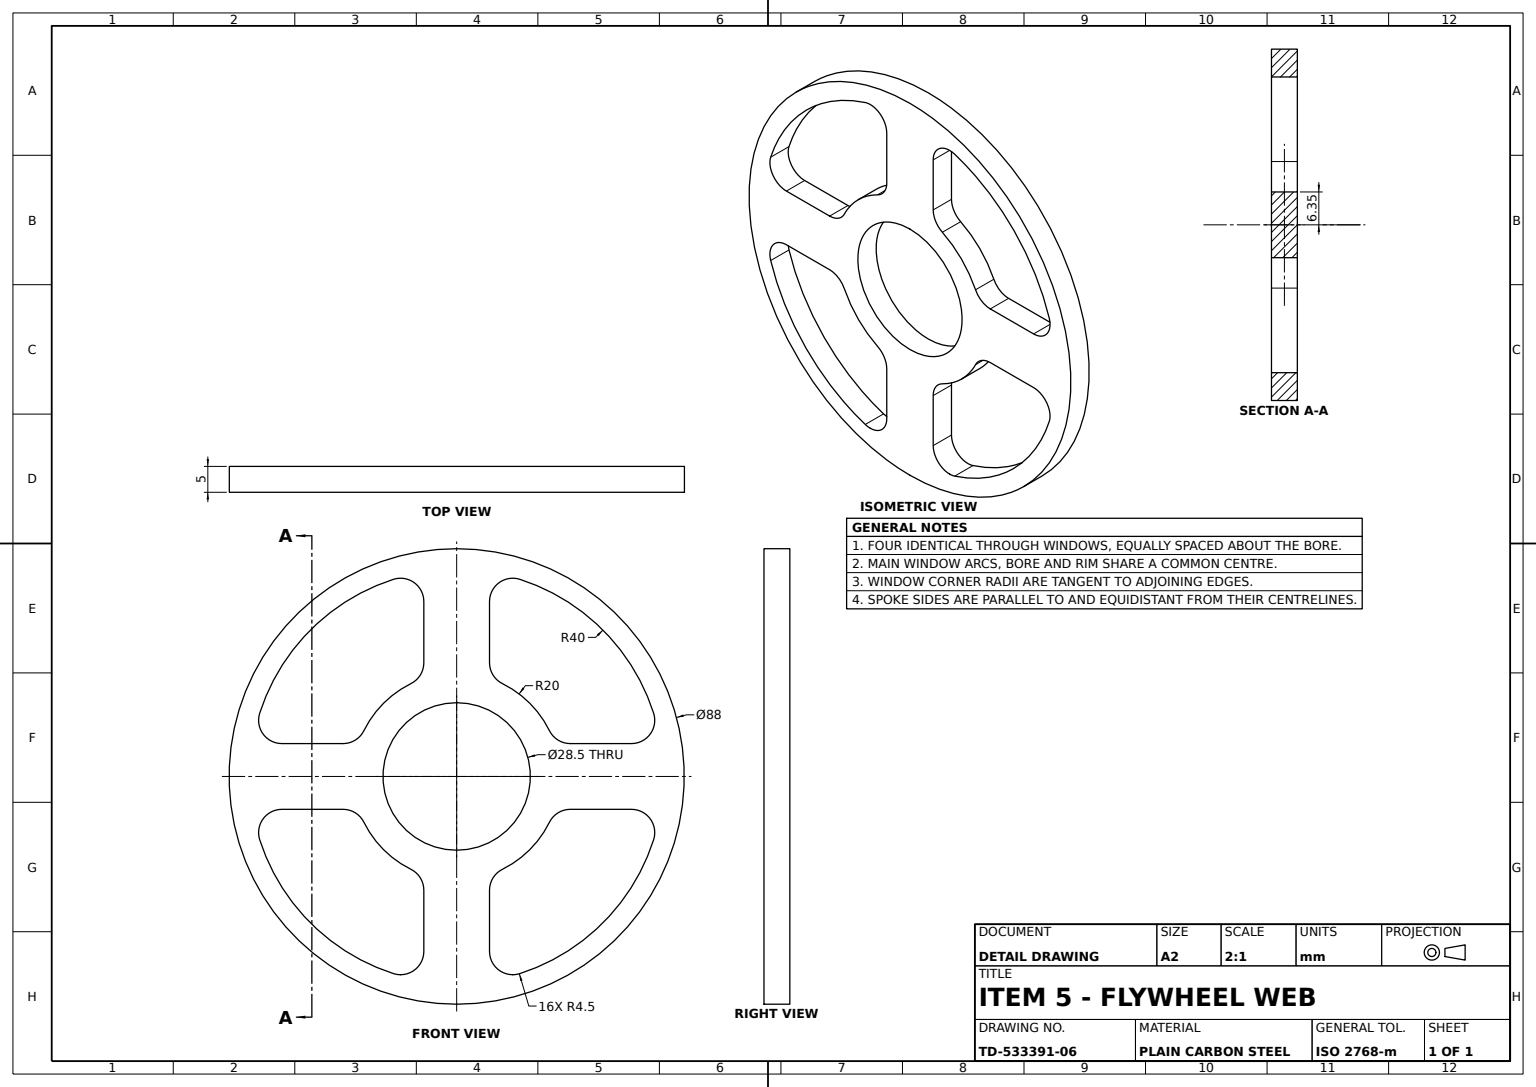
ISO-10303-21;
HEADER;
FILE_DESCRIPTION((''),'2;1');
FILE_NAME('','',(''),(''),'','','');
FILE_SCHEMA(('AUTOMOTIVE_DESIGN'));
ENDSEC;
DATA;
#1=APPLICATION_CONTEXT('');
#2=PRODUCT_CONTEXT('',#1,'mechanical');
#3=PRODUCT('','','',(#2));
#4=PRODUCT_DEFINITION_FORMATION('','',#3);
#5=PRODUCT_DEFINITION_CONTEXT('',#1,'design');
#6=PRODUCT_DEFINITION('','',#4,#5);
#7=PRODUCT_DEFINITION_SHAPE('','',#6);
#8=(LENGTH_UNIT()NAMED_UNIT(*)SI_UNIT(.MILLI.,.METRE.));
#9=(NAMED_UNIT(*)PLANE_ANGLE_UNIT()SI_UNIT($,.RADIAN.));
#10=(NAMED_UNIT(*)SI_UNIT($,.STERADIAN.)SOLID_ANGLE_UNIT());
#11=UNCERTAINTY_MEASURE_WITH_UNIT(LENGTH_MEASURE(1.E-05),#8,'distance_accuracy_value','');
#12=(GEOMETRIC_REPRESENTATION_CONTEXT(3)GLOBAL_UNCERTAINTY_ASSIGNED_CONTEXT((#11))GLOBAL_UNIT_ASSIGNED_CONTEXT((#8,#9,#10))REPRESENTATION_CONTEXT('',''));
#13=CARTESIAN_POINT('',(12.225352,0.,38.085965));
#14=VERTEX_POINT('',#13);
#15=CARTESIAN_POINT('',(12.225352,5.,38.085965));
#16=VERTEX_POINT('',#15);
#17=CARTESIAN_POINT('',(12.225352,-39.,38.085965));
#18=DIRECTION('',(0.,1.,0.));
#19=VECTOR('',#18,1000.);
#20=LINE('',#17,#19);
#21=EDGE_CURVE('',#14,#16,#20,.T.);
#22=ORIENTED_EDGE('',*,*,#21,.T.);
#23=CARTESIAN_POINT('',(38.085965,5.,12.225352));
#24=VERTEX_POINT('',#23);
#25=CARTESIAN_POINT('',(0.,5.,0.));
#26=DIRECTION('',(0.,0.,1.));
#27=AXIS2_PLACEMENT_3D('',#25,#18,#26);
#28=CIRCLE('',#27,40.);
#29=EDGE_CURVE('',#16,#24,#28,.T.);
#30=ORIENTED_EDGE('',*,*,#29,.T.);
#31=CARTESIAN_POINT('',(38.085965,0.,12.225352));
#32=VERTEX_POINT('',#31);
#33=CARTESIAN_POINT('',(38.085965,-39.,12.225352));
#34=LINE('',#33,#19);
#35=EDGE_CURVE('',#32,#24,#34,.T.);
#36=ORIENTED_EDGE('',*,*,#35,.F.);
#37=CARTESIAN_POINT('',(0.,0.,0.));
#38=AXIS2_PLACEMENT_3D('',#37,#18,#26);
#39=CIRCLE('',#38,40.);
#40=EDGE_CURVE('',#14,#32,#39,.T.);
#41=ORIENTED_EDGE('',*,*,#40,.F.);
#42=EDGE_LOOP('',(#22,#30,#36,#41));
#43=FACE_OUTER_BOUND('',#42,.T.);
#44=CARTESIAN_POINT('',(0.,-39.,0.));
#45=AXIS2_PLACEMENT_3D('',#44,#18,#26);
#46=CYLINDRICAL_SURFACE('',#45,40.);
#47=ADVANCED_FACE('',(#43),#46,.F.);
#48=CARTESIAN_POINT('',(0.,5.,-44.));
#49=VERTEX_POINT('',#48);
#50=CARTESIAN_POINT('',(0.,0.,-44.));
#51=VERTEX_POINT('',#50);
#52=DIRECTION('',(0.,-1.,0.));
#53=VECTOR('',#52,1000.);
#54=LINE('',#48,#53);
#55=EDGE_CURVE('',#49,#51,#54,.T.);
#56=ORIENTED_EDGE('',*,*,#55,.F.);
#57=CARTESIAN_POINT('',(0.,5.,44.));
#58=VERTEX_POINT('',#57);
#59=CIRCLE('',#27,44.);
#60=EDGE_CURVE('',#58,#49,#59,.T.);
#61=ORIENTED_EDGE('',*,*,#60,.F.);
#62=CARTESIAN_POINT('',(0.,0.,44.));
#63=VERTEX_POINT('',#62);
#64=LINE('',#57,#53);
#65=EDGE_CURVE('',#58,#63,#64,.T.);
#66=ORIENTED_EDGE('',*,*,#65,.T.);
#67=CIRCLE('',#38,44.);
#68=EDGE_CURVE('',#63,#51,#67,.T.);
#69=ORIENTED_EDGE('',*,*,#68,.T.);
#70=EDGE_LOOP('',(#56,#61,#66,#69));
#71=FACE_OUTER_BOUND('',#70,.T.);
#72=DIRECTION('',(0.,0.,-1.));
#73=AXIS2_PLACEMENT_3D('',#25,#52,#72);
#74=CYLINDRICAL_SURFACE('',#73,44.);
#75=ADVANCED_FACE('',(#71),#74,.T.);
#76=CARTESIAN_POINT('',(10.85,0.,38.301294));
#77=VERTEX_POINT('',#76);
#78=CARTESIAN_POINT('',(10.85,5.,38.301294));
#79=VERTEX_POINT('',#78);
#80=CARTESIAN_POINT('',(10.85,-39.,38.301294));
#81=LINE('',#80,#19);
#82=EDGE_CURVE('',#77,#79,#81,.T.);
#83=ORIENTED_EDGE('',*,*,#82,.T.);
#84=CARTESIAN_POINT('',(10.85,5.,33.801294));
#85=AXIS2_PLACEMENT_3D('',#84,#18,#26);
#86=CIRCLE('',#85,4.5);
#87=EDGE_CURVE('',#79,#16,#86,.T.);
#88=ORIENTED_EDGE('',*,*,#87,.T.);
#89=ORIENTED_EDGE('',*,*,#21,.F.);
#90=CARTESIAN_POINT('',(10.85,0.,33.801294));
#91=AXIS2_PLACEMENT_3D('',#90,#18,#26);
#92=CIRCLE('',#91,4.5);
#93=EDGE_CURVE('',#77,#14,#92,.T.);
#94=ORIENTED_EDGE('',*,*,#93,.F.);
#95=EDGE_LOOP('',(#83,#88,#89,#94));
#96=FACE_OUTER_BOUND('',#95,.T.);
#97=CARTESIAN_POINT('',(10.85,-39.,33.801294));
#98=AXIS2_PLACEMENT_3D('',#97,#18,#26);
#99=CYLINDRICAL_SURFACE('',#98,4.5);
#100=ADVANCED_FACE('',(#96),#99,.F.);
#101=CARTESIAN_POINT('',(-8.857143,0.,17.931844));
#102=VERTEX_POINT('',#101);
#103=CARTESIAN_POINT('',(-8.857143,5.,17.931844));
#104=VERTEX_POINT('',#103);
#105=CARTESIAN_POINT('',(-8.857143,-39.,17.931844));
#106=LINE('',#105,#19);
#107=EDGE_CURVE('',#102,#104,#106,.T.);
#108=ORIENTED_EDGE('',*,*,#107,.F.);
#109=CARTESIAN_POINT('',(-6.35,0.,21.966509));
#110=VERTEX_POINT('',#109);
#111=CARTESIAN_POINT('',(-10.85,0.,21.966509));
#112=AXIS2_PLACEMENT_3D('',#111,#18,#26);
#113=CIRCLE('',#112,4.5);
#114=EDGE_CURVE('',#110,#102,#113,.T.);
#115=ORIENTED_EDGE('',*,*,#114,.F.);
#116=CARTESIAN_POINT('',(-6.35,5.,21.966509));
#117=VERTEX_POINT('',#116);
#118=CARTESIAN_POINT('',(-6.35,-39.,21.966509));
#119=LINE('',#118,#19);
#120=EDGE_CURVE('',#110,#117,#119,.T.);
#121=ORIENTED_EDGE('',*,*,#120,.T.);
#122=CARTESIAN_POINT('',(-10.85,5.,21.966509));
#123=AXIS2_PLACEMENT_3D('',#122,#18,#26);
#124=CIRCLE('',#123,4.5);
#125=EDGE_CURVE('',#117,#104,#124,.T.);
#126=ORIENTED_EDGE('',*,*,#125,.T.);
#127=EDGE_LOOP('',(#108,#115,#121,#126));
#128=FACE_OUTER_BOUND('',#127,.T.);
#129=CARTESIAN_POINT('',(-10.85,-39.,21.966509));
#130=AXIS2_PLACEMENT_3D('',#129,#18,#26);
#131=CYLINDRICAL_SURFACE('',#130,4.5);
#132=ADVANCED_FACE('',(#128),#131,.F.);
#133=CARTESIAN_POINT('',(-17.931844,0.,8.857143));
#134=VERTEX_POINT('',#133);
#135=CIRCLE('',#38,20.);
#136=EDGE_CURVE('',#134,#102,#135,.T.);
#137=ORIENTED_EDGE('',*,*,#136,.F.);
#138=CARTESIAN_POINT('',(-21.966509,0.,6.35));
#139=VERTEX_POINT('',#138);
#140=CARTESIAN_POINT('',(-21.966509,0.,10.85));
#141=AXIS2_PLACEMENT_3D('',#140,#18,#26);
#142=CIRCLE('',#141,4.5);
#143=EDGE_CURVE('',#134,#139,#142,.T.);
#144=ORIENTED_EDGE('',*,*,#143,.T.);
#145=CARTESIAN_POINT('',(-33.801294,0.,6.35));
#146=VERTEX_POINT('',#145);
#147=CARTESIAN_POINT('',(0.,0.,6.35));
#148=DIRECTION('',(-1.,0.,0.));
#149=VECTOR('',#148,1000.);
#150=LINE('',#147,#149);
#151=EDGE_CURVE('',#139,#146,#150,.T.);
#152=ORIENTED_EDGE('',*,*,#151,.T.);
#153=CARTESIAN_POINT('',(-38.085965,0.,12.225352));
#154=VERTEX_POINT('',#153);
#155=CARTESIAN_POINT('',(-33.801294,0.,10.85));
#156=AXIS2_PLACEMENT_3D('',#155,#18,#26);
#157=CIRCLE('',#156,4.5);
#158=EDGE_CURVE('',#146,#154,#157,.T.);
#159=ORIENTED_EDGE('',*,*,#158,.T.);
#160=CARTESIAN_POINT('',(-12.225352,0.,38.085965));
#161=VERTEX_POINT('',#160);
#162=EDGE_CURVE('',#154,#161,#39,.T.);
#163=ORIENTED_EDGE('',*,*,#162,.T.);
#164=CARTESIAN_POINT('',(-10.85,0.,38.301294));
#165=VERTEX_POINT('',#164);
#166=CARTESIAN_POINT('',(-10.85,0.,33.801294));
#167=AXIS2_PLACEMENT_3D('',#166,#18,#26);
#168=CIRCLE('',#167,4.5);
#169=EDGE_CURVE('',#161,#165,#168,.T.);
#170=ORIENTED_EDGE('',*,*,#169,.T.);
#171=CARTESIAN_POINT('',(-6.35,0.,33.801294));
#172=VERTEX_POINT('',#171);
#173=EDGE_CURVE('',#165,#172,#168,.T.);
#174=ORIENTED_EDGE('',*,*,#173,.T.);
#175=CARTESIAN_POINT('',(-6.35,0.,0.));
#176=VECTOR('',#26,1000.);
#177=LINE('',#175,#176);
#178=EDGE_CURVE('',#110,#172,#177,.T.);
#179=ORIENTED_EDGE('',*,*,#178,.F.);
#180=ORIENTED_EDGE('',*,*,#114,.T.);
#181=EDGE_LOOP('',(#137,#144,#152,#159,#163,#170,#174,#179,#180));
#182=FACE_BOUND('',#181,.T.);
#183=CARTESIAN_POINT('',(6.35,0.,33.801294));
#184=VERTEX_POINT('',#183);
#185=EDGE_CURVE('',#184,#77,#92,.T.);
#186=ORIENTED_EDGE('',*,*,#185,.T.);
#187=ORIENTED_EDGE('',*,*,#93,.T.);
#188=ORIENTED_EDGE('',*,*,#40,.T.);
#189=CARTESIAN_POINT('',(33.801294,0.,6.35));
#190=VERTEX_POINT('',#189);
#191=CARTESIAN_POINT('',(33.801294,0.,10.85));
#192=AXIS2_PLACEMENT_3D('',#191,#18,#26);
#193=CIRCLE('',#192,4.5);
#194=EDGE_CURVE('',#32,#190,#193,.T.);
#195=ORIENTED_EDGE('',*,*,#194,.T.);
#196=CARTESIAN_POINT('',(21.966509,0.,6.35));
#197=VERTEX_POINT('',#196);
#198=DIRECTION('',(1.,0.,0.));
#199=VECTOR('',#198,1000.);
#200=LINE('',#147,#199);
#201=EDGE_CURVE('',#197,#190,#200,.T.);
#202=ORIENTED_EDGE('',*,*,#201,.F.);
#203=CARTESIAN_POINT('',(17.931844,0.,8.857143));
#204=VERTEX_POINT('',#203);
#205=CARTESIAN_POINT('',(21.966509,0.,10.85));
#206=AXIS2_PLACEMENT_3D('',#205,#18,#26);
#207=CIRCLE('',#206,4.5);
#208=EDGE_CURVE('',#197,#204,#207,.T.);
#209=ORIENTED_EDGE('',*,*,#208,.T.);
#210=CARTESIAN_POINT('',(8.857143,0.,17.931844));
#211=VERTEX_POINT('',#210);
#212=EDGE_CURVE('',#211,#204,#135,.T.);
#213=ORIENTED_EDGE('',*,*,#212,.F.);
#214=CARTESIAN_POINT('',(6.35,0.,21.966509));
#215=VERTEX_POINT('',#214);
#216=CARTESIAN_POINT('',(10.85,0.,21.966509));
#217=AXIS2_PLACEMENT_3D('',#216,#18,#26);
#218=CIRCLE('',#217,4.5);
#219=EDGE_CURVE('',#211,#215,#218,.T.);
#220=ORIENTED_EDGE('',*,*,#219,.T.);
#221=CARTESIAN_POINT('',(6.35,0.,0.));
#222=LINE('',#221,#176);
#223=EDGE_CURVE('',#215,#184,#222,.T.);
#224=ORIENTED_EDGE('',*,*,#223,.T.);
#225=EDGE_LOOP('',(#186,#187,#188,#195,#202,#209,#213,#220,#224));
#226=FACE_BOUND('',#225,.T.);
#227=CARTESIAN_POINT('',(0.,0.,14.25));
#228=VERTEX_POINT('',#227);
#229=CARTESIAN_POINT('',(0.,0.,-14.25));
#230=VERTEX_POINT('',#229);
#231=CIRCLE('',#38,14.25);
#232=EDGE_CURVE('',#228,#230,#231,.T.);
#233=ORIENTED_EDGE('',*,*,#232,.T.);
#234=EDGE_CURVE('',#230,#228,#231,.T.);
#235=ORIENTED_EDGE('',*,*,#234,.T.);
#236=EDGE_LOOP('',(#233,#235));
#237=FACE_BOUND('',#236,.T.);
#238=CARTESIAN_POINT('',(-12.225352,0.,-38.085965));
#239=VERTEX_POINT('',#238);
#240=CARTESIAN_POINT('',(-38.085965,0.,-12.225352));
#241=VERTEX_POINT('',#240);
#242=EDGE_CURVE('',#239,#241,#39,.T.);
#243=ORIENTED_EDGE('',*,*,#242,.T.);
#244=CARTESIAN_POINT('',(-33.801294,0.,-6.35));
#245=VERTEX_POINT('',#244);
#246=CARTESIAN_POINT('',(-33.801294,0.,-10.85));
#247=AXIS2_PLACEMENT_3D('',#246,#18,#26);
#248=CIRCLE('',#247,4.5);
#249=EDGE_CURVE('',#241,#245,#248,.T.);
#250=ORIENTED_EDGE('',*,*,#249,.T.);
#251=CARTESIAN_POINT('',(-21.966509,0.,-6.35));
#252=VERTEX_POINT('',#251);
#253=CARTESIAN_POINT('',(0.,0.,-6.35));
#254=LINE('',#253,#149);
#255=EDGE_CURVE('',#252,#245,#254,.T.);
#256=ORIENTED_EDGE('',*,*,#255,.F.);
#257=CARTESIAN_POINT('',(-17.931844,0.,-8.857143));
#258=VERTEX_POINT('',#257);
#259=CARTESIAN_POINT('',(-21.966509,0.,-10.85));
#260=AXIS2_PLACEMENT_3D('',#259,#18,#26);
#261=CIRCLE('',#260,4.5);
#262=EDGE_CURVE('',#252,#258,#261,.T.);
#263=ORIENTED_EDGE('',*,*,#262,.T.);
#264=CARTESIAN_POINT('',(-8.857143,0.,-17.931844));
#265=VERTEX_POINT('',#264);
#266=EDGE_CURVE('',#265,#258,#135,.T.);
#267=ORIENTED_EDGE('',*,*,#266,.F.);
#268=CARTESIAN_POINT('',(-6.35,0.,-21.966509));
#269=VERTEX_POINT('',#268);
#270=CARTESIAN_POINT('',(-10.85,0.,-21.966509));
#271=AXIS2_PLACEMENT_3D('',#270,#18,#26);
#272=CIRCLE('',#271,4.5);
#273=EDGE_CURVE('',#265,#269,#272,.T.);
#274=ORIENTED_EDGE('',*,*,#273,.T.);
#275=CARTESIAN_POINT('',(-6.35,0.,-33.801294));
#276=VERTEX_POINT('',#275);
#277=VECTOR('',#72,1000.);
#278=LINE('',#175,#277);
#279=EDGE_CURVE('',#269,#276,#278,.T.);
#280=ORIENTED_EDGE('',*,*,#279,.T.);
#281=CARTESIAN_POINT('',(-10.85,0.,-33.801294));
#282=AXIS2_PLACEMENT_3D('',#281,#18,#26);
#283=CIRCLE('',#282,4.5);
#284=EDGE_CURVE('',#276,#239,#283,.T.);
#285=ORIENTED_EDGE('',*,*,#284,.T.);
#286=EDGE_LOOP('',(#243,#250,#256,#263,#267,#274,#280,#285));
#287=FACE_BOUND('',#286,.T.);
#288=CARTESIAN_POINT('',(6.35,0.,-21.966509));
#289=VERTEX_POINT('',#288);
#290=CARTESIAN_POINT('',(6.35,0.,-33.801294));
#291=VERTEX_POINT('',#290);
#292=LINE('',#221,#277);
#293=EDGE_CURVE('',#289,#291,#292,.T.);
#294=ORIENTED_EDGE('',*,*,#293,.F.);
#295=CARTESIAN_POINT('',(8.857143,0.,-17.931844));
#296=VERTEX_POINT('',#295);
#297=CARTESIAN_POINT('',(10.85,0.,-21.966509));
#298=AXIS2_PLACEMENT_3D('',#297,#18,#26);
#299=CIRCLE('',#298,4.5);
#300=EDGE_CURVE('',#289,#296,#299,.T.);
#301=ORIENTED_EDGE('',*,*,#300,.T.);
#302=CARTESIAN_POINT('',(17.931844,0.,-8.857143));
#303=VERTEX_POINT('',#302);
#304=EDGE_CURVE('',#303,#296,#135,.T.);
#305=ORIENTED_EDGE('',*,*,#304,.F.);
#306=CARTESIAN_POINT('',(21.966509,0.,-6.35));
#307=VERTEX_POINT('',#306);
#308=CARTESIAN_POINT('',(21.966509,0.,-10.85));
#309=AXIS2_PLACEMENT_3D('',#308,#18,#26);
#310=CIRCLE('',#309,4.5);
#311=EDGE_CURVE('',#303,#307,#310,.T.);
#312=ORIENTED_EDGE('',*,*,#311,.T.);
#313=CARTESIAN_POINT('',(33.801294,0.,-6.35));
#314=VERTEX_POINT('',#313);
#315=LINE('',#253,#199);
#316=EDGE_CURVE('',#307,#314,#315,.T.);
#317=ORIENTED_EDGE('',*,*,#316,.T.);
#318=CARTESIAN_POINT('',(38.085965,0.,-12.225352));
#319=VERTEX_POINT('',#318);
#320=CARTESIAN_POINT('',(33.801294,0.,-10.85));
#321=AXIS2_PLACEMENT_3D('',#320,#18,#26);
#322=CIRCLE('',#321,4.5);
#323=EDGE_CURVE('',#314,#319,#322,.T.);
#324=ORIENTED_EDGE('',*,*,#323,.T.);
#325=CARTESIAN_POINT('',(12.225352,0.,-38.085965));
#326=VERTEX_POINT('',#325);
#327=EDGE_CURVE('',#319,#326,#39,.T.);
#328=ORIENTED_EDGE('',*,*,#327,.T.);
#329=CARTESIAN_POINT('',(10.85,0.,-33.801294));
#330=AXIS2_PLACEMENT_3D('',#329,#18,#26);
#331=CIRCLE('',#330,4.5);
#332=EDGE_CURVE('',#326,#291,#331,.T.);
#333=ORIENTED_EDGE('',*,*,#332,.T.);
#334=EDGE_LOOP('',(#294,#301,#305,#312,#317,#324,#328,#333));
#335=FACE_BOUND('',#334,.T.);
#336=EDGE_CURVE('',#51,#63,#67,.T.);
#337=ORIENTED_EDGE('',*,*,#336,.F.);
#338=ORIENTED_EDGE('',*,*,#68,.F.);
#339=EDGE_LOOP('',(#337,#338));
#340=FACE_OUTER_BOUND('',#339,.T.);
#341=PLANE('',#38);
#342=ADVANCED_FACE('',(#182,#226,#237,#287,#335,#340),#341,.F.);
#343=CARTESIAN_POINT('',(-8.857143,5.,-17.931844));
#344=VERTEX_POINT('',#343);
#345=CARTESIAN_POINT('',(-6.35,5.,-21.966509));
#346=VERTEX_POINT('',#345);
#347=CARTESIAN_POINT('',(-10.85,5.,-21.966509));
#348=AXIS2_PLACEMENT_3D('',#347,#18,#26);
#349=CIRCLE('',#348,4.5);
#350=EDGE_CURVE('',#344,#346,#349,.T.);
#351=ORIENTED_EDGE('',*,*,#350,.F.);
#352=CARTESIAN_POINT('',(-17.931844,5.,-8.857143));
#353=VERTEX_POINT('',#352);
#354=CIRCLE('',#27,20.);
#355=EDGE_CURVE('',#344,#353,#354,.T.);
#356=ORIENTED_EDGE('',*,*,#355,.T.);
#357=CARTESIAN_POINT('',(-21.966509,5.,-6.35));
#358=VERTEX_POINT('',#357);
#359=CARTESIAN_POINT('',(-21.966509,5.,-10.85));
#360=AXIS2_PLACEMENT_3D('',#359,#18,#26);
#361=CIRCLE('',#360,4.5);
#362=EDGE_CURVE('',#358,#353,#361,.T.);
#363=ORIENTED_EDGE('',*,*,#362,.F.);
#364=CARTESIAN_POINT('',(-33.801294,5.,-6.35));
#365=VERTEX_POINT('',#364);
#366=CARTESIAN_POINT('',(0.,5.,-6.35));
#367=LINE('',#366,#149);
#368=EDGE_CURVE('',#358,#365,#367,.T.);
#369=ORIENTED_EDGE('',*,*,#368,.T.);
#370=CARTESIAN_POINT('',(-38.085965,5.,-12.225352));
#371=VERTEX_POINT('',#370);
#372=CARTESIAN_POINT('',(-33.801294,5.,-10.85));
#373=AXIS2_PLACEMENT_3D('',#372,#18,#26);
#374=CIRCLE('',#373,4.5);
#375=EDGE_CURVE('',#371,#365,#374,.T.);
#376=ORIENTED_EDGE('',*,*,#375,.F.);
#377=CARTESIAN_POINT('',(-12.225352,5.,-38.085965));
#378=VERTEX_POINT('',#377);
#379=EDGE_CURVE('',#378,#371,#28,.T.);
#380=ORIENTED_EDGE('',*,*,#379,.F.);
#381=CARTESIAN_POINT('',(-6.35,5.,-33.801294));
#382=VERTEX_POINT('',#381);
#383=CARTESIAN_POINT('',(-10.85,5.,-33.801294));
#384=AXIS2_PLACEMENT_3D('',#383,#18,#26);
#385=CIRCLE('',#384,4.5);
#386=EDGE_CURVE('',#382,#378,#385,.T.);
#387=ORIENTED_EDGE('',*,*,#386,.F.);
#388=CARTESIAN_POINT('',(-6.35,5.,0.));
#389=LINE('',#388,#277);
#390=EDGE_CURVE('',#346,#382,#389,.T.);
#391=ORIENTED_EDGE('',*,*,#390,.F.);
#392=EDGE_LOOP('',(#351,#356,#363,#369,#376,#380,#387,#391));
#393=FACE_BOUND('',#392,.T.);
#394=CARTESIAN_POINT('',(6.35,5.,-21.966509));
#395=VERTEX_POINT('',#394);
#396=CARTESIAN_POINT('',(8.857143,5.,-17.931844));
#397=VERTEX_POINT('',#396);
#398=CARTESIAN_POINT('',(10.85,5.,-21.966509));
#399=AXIS2_PLACEMENT_3D('',#398,#18,#26);
#400=CIRCLE('',#399,4.5);
#401=EDGE_CURVE('',#395,#397,#400,.T.);
#402=ORIENTED_EDGE('',*,*,#401,.F.);
#403=CARTESIAN_POINT('',(6.35,5.,-33.801294));
#404=VERTEX_POINT('',#403);
#405=CARTESIAN_POINT('',(6.35,5.,0.));
#406=LINE('',#405,#277);
#407=EDGE_CURVE('',#395,#404,#406,.T.);
#408=ORIENTED_EDGE('',*,*,#407,.T.);
#409=CARTESIAN_POINT('',(12.225352,5.,-38.085965));
#410=VERTEX_POINT('',#409);
#411=CARTESIAN_POINT('',(10.85,5.,-33.801294));
#412=AXIS2_PLACEMENT_3D('',#411,#18,#26);
#413=CIRCLE('',#412,4.5);
#414=EDGE_CURVE('',#410,#404,#413,.T.);
#415=ORIENTED_EDGE('',*,*,#414,.F.);
#416=CARTESIAN_POINT('',(38.085965,5.,-12.225352));
#417=VERTEX_POINT('',#416);
#418=EDGE_CURVE('',#417,#410,#28,.T.);
#419=ORIENTED_EDGE('',*,*,#418,.F.);
#420=CARTESIAN_POINT('',(33.801294,5.,-6.35));
#421=VERTEX_POINT('',#420);
#422=CARTESIAN_POINT('',(33.801294,5.,-10.85));
#423=AXIS2_PLACEMENT_3D('',#422,#18,#26);
#424=CIRCLE('',#423,4.5);
#425=EDGE_CURVE('',#421,#417,#424,.T.);
#426=ORIENTED_EDGE('',*,*,#425,.F.);
#427=CARTESIAN_POINT('',(21.966509,5.,-6.35));
#428=VERTEX_POINT('',#427);
#429=LINE('',#366,#199);
#430=EDGE_CURVE('',#428,#421,#429,.T.);
#431=ORIENTED_EDGE('',*,*,#430,.F.);
#432=CARTESIAN_POINT('',(17.931844,5.,-8.857143));
#433=VERTEX_POINT('',#432);
#434=CARTESIAN_POINT('',(21.966509,5.,-10.85));
#435=AXIS2_PLACEMENT_3D('',#434,#18,#26);
#436=CIRCLE('',#435,4.5);
#437=EDGE_CURVE('',#433,#428,#436,.T.);
#438=ORIENTED_EDGE('',*,*,#437,.F.);
#439=EDGE_CURVE('',#433,#397,#354,.T.);
#440=ORIENTED_EDGE('',*,*,#439,.T.);
#441=EDGE_LOOP('',(#402,#408,#415,#419,#426,#431,#438,#440));
#442=FACE_BOUND('',#441,.T.);
#443=CARTESIAN_POINT('',(21.966509,5.,6.35));
#444=VERTEX_POINT('',#443);
#445=CARTESIAN_POINT('',(33.801294,5.,6.35));
#446=VERTEX_POINT('',#445);
#447=CARTESIAN_POINT('',(0.,5.,6.35));
#448=LINE('',#447,#199);
#449=EDGE_CURVE('',#444,#446,#448,.T.);
#450=ORIENTED_EDGE('',*,*,#449,.T.);
#451=CARTESIAN_POINT('',(33.801294,5.,10.85));
#452=AXIS2_PLACEMENT_3D('',#451,#18,#26);
#453=CIRCLE('',#452,4.5);
#454=EDGE_CURVE('',#24,#446,#453,.T.);
#455=ORIENTED_EDGE('',*,*,#454,.F.);
#456=ORIENTED_EDGE('',*,*,#29,.F.);
#457=ORIENTED_EDGE('',*,*,#87,.F.);
#458=CARTESIAN_POINT('',(6.35,5.,33.801294));
#459=VERTEX_POINT('',#458);
#460=EDGE_CURVE('',#459,#79,#86,.T.);
#461=ORIENTED_EDGE('',*,*,#460,.F.);
#462=CARTESIAN_POINT('',(6.35,5.,21.966509));
#463=VERTEX_POINT('',#462);
#464=LINE('',#405,#176);
#465=EDGE_CURVE('',#463,#459,#464,.T.);
#466=ORIENTED_EDGE('',*,*,#465,.F.);
#467=CARTESIAN_POINT('',(8.857143,5.,17.931844));
#468=VERTEX_POINT('',#467);
#469=CARTESIAN_POINT('',(10.85,5.,21.966509));
#470=AXIS2_PLACEMENT_3D('',#469,#18,#26);
#471=CIRCLE('',#470,4.5);
#472=EDGE_CURVE('',#468,#463,#471,.T.);
#473=ORIENTED_EDGE('',*,*,#472,.F.);
#474=CARTESIAN_POINT('',(17.931844,5.,8.857143));
#475=VERTEX_POINT('',#474);
#476=EDGE_CURVE('',#468,#475,#354,.T.);
#477=ORIENTED_EDGE('',*,*,#476,.T.);
#478=CARTESIAN_POINT('',(21.966509,5.,10.85));
#479=AXIS2_PLACEMENT_3D('',#478,#18,#26);
#480=CIRCLE('',#479,4.5);
#481=EDGE_CURVE('',#444,#475,#480,.T.);
#482=ORIENTED_EDGE('',*,*,#481,.F.);
#483=EDGE_LOOP('',(#450,#455,#456,#457,#461,#466,#473,#477,#482));
#484=FACE_BOUND('',#483,.T.);
#485=ORIENTED_EDGE('',*,*,#60,.T.);
#486=EDGE_CURVE('',#49,#58,#59,.T.);
#487=ORIENTED_EDGE('',*,*,#486,.T.);
#488=EDGE_LOOP('',(#485,#487));
#489=FACE_OUTER_BOUND('',#488,.T.);
#490=CARTESIAN_POINT('',(-17.931844,5.,8.857143));
#491=VERTEX_POINT('',#490);
#492=CARTESIAN_POINT('',(-21.966509,5.,6.35));
#493=VERTEX_POINT('',#492);
#494=CARTESIAN_POINT('',(-21.966509,5.,10.85));
#495=AXIS2_PLACEMENT_3D('',#494,#18,#26);
#496=CIRCLE('',#495,4.5);
#497=EDGE_CURVE('',#491,#493,#496,.T.);
#498=ORIENTED_EDGE('',*,*,#497,.F.);
#499=EDGE_CURVE('',#491,#104,#354,.T.);
#500=ORIENTED_EDGE('',*,*,#499,.T.);
#501=ORIENTED_EDGE('',*,*,#125,.F.);
#502=CARTESIAN_POINT('',(-6.35,5.,33.801294));
#503=VERTEX_POINT('',#502);
#504=LINE('',#388,#176);
#505=EDGE_CURVE('',#117,#503,#504,.T.);
#506=ORIENTED_EDGE('',*,*,#505,.T.);
#507=CARTESIAN_POINT('',(-10.85,5.,38.301294));
#508=VERTEX_POINT('',#507);
#509=CARTESIAN_POINT('',(-10.85,5.,33.801294));
#510=AXIS2_PLACEMENT_3D('',#509,#18,#26);
#511=CIRCLE('',#510,4.5);
#512=EDGE_CURVE('',#508,#503,#511,.T.);
#513=ORIENTED_EDGE('',*,*,#512,.F.);
#514=CARTESIAN_POINT('',(-12.225352,5.,38.085965));
#515=VERTEX_POINT('',#514);
#516=EDGE_CURVE('',#515,#508,#511,.T.);
#517=ORIENTED_EDGE('',*,*,#516,.F.);
#518=CARTESIAN_POINT('',(-38.085965,5.,12.225352));
#519=VERTEX_POINT('',#518);
#520=EDGE_CURVE('',#519,#515,#28,.T.);
#521=ORIENTED_EDGE('',*,*,#520,.F.);
#522=CARTESIAN_POINT('',(-33.801294,5.,6.35));
#523=VERTEX_POINT('',#522);
#524=CARTESIAN_POINT('',(-33.801294,5.,10.85));
#525=AXIS2_PLACEMENT_3D('',#524,#18,#26);
#526=CIRCLE('',#525,4.5);
#527=EDGE_CURVE('',#523,#519,#526,.T.);
#528=ORIENTED_EDGE('',*,*,#527,.F.);
#529=LINE('',#447,#149);
#530=EDGE_CURVE('',#493,#523,#529,.T.);
#531=ORIENTED_EDGE('',*,*,#530,.F.);
#532=EDGE_LOOP('',(#498,#500,#501,#506,#513,#517,#521,#528,#531));
#533=FACE_BOUND('',#532,.T.);
#534=CARTESIAN_POINT('',(0.,5.,14.25));
#535=VERTEX_POINT('',#534);
#536=CARTESIAN_POINT('',(0.,5.,-14.25));
#537=VERTEX_POINT('',#536);
#538=CIRCLE('',#27,14.25);
#539=EDGE_CURVE('',#535,#537,#538,.T.);
#540=ORIENTED_EDGE('',*,*,#539,.F.);
#541=EDGE_CURVE('',#537,#535,#538,.T.);
#542=ORIENTED_EDGE('',*,*,#541,.F.);
#543=EDGE_LOOP('',(#540,#542));
#544=FACE_BOUND('',#543,.T.);
#545=PLANE('',#27);
#546=ADVANCED_FACE('',(#393,#442,#484,#489,#533,#544),#545,.T.);
#547=CARTESIAN_POINT('',(-6.35,-39.,-21.966509));
#548=LINE('',#547,#19);
#549=EDGE_CURVE('',#269,#346,#548,.T.);
#550=ORIENTED_EDGE('',*,*,#549,.T.);
#551=ORIENTED_EDGE('',*,*,#390,.T.);
#552=CARTESIAN_POINT('',(-6.35,-39.,-33.801294));
#553=LINE('',#552,#19);
#554=EDGE_CURVE('',#276,#382,#553,.T.);
#555=ORIENTED_EDGE('',*,*,#554,.F.);
#556=ORIENTED_EDGE('',*,*,#279,.F.);
#557=EDGE_LOOP('',(#550,#551,#555,#556));
#558=FACE_OUTER_BOUND('',#557,.T.);
#559=CARTESIAN_POINT('',(-6.35,-39.,0.));
#560=AXIS2_PLACEMENT_3D('',#559,#198,#72);
#561=PLANE('',#560);
#562=ADVANCED_FACE('',(#558),#561,.F.);
#563=ORIENTED_EDGE('',*,*,#355,.F.);
#564=CARTESIAN_POINT('',(-8.857143,-39.,-17.931844));
#565=LINE('',#564,#19);
#566=EDGE_CURVE('',#265,#344,#565,.T.);
#567=ORIENTED_EDGE('',*,*,#566,.F.);
#568=ORIENTED_EDGE('',*,*,#266,.T.);
#569=CARTESIAN_POINT('',(-17.931844,-39.,-8.857143));
#570=LINE('',#569,#19);
#571=EDGE_CURVE('',#258,#353,#570,.T.);
#572=ORIENTED_EDGE('',*,*,#571,.T.);
#573=EDGE_LOOP('',(#563,#567,#568,#572));
#574=FACE_OUTER_BOUND('',#573,.T.);
#575=CYLINDRICAL_SURFACE('',#45,20.);
#576=ADVANCED_FACE('',(#574),#575,.T.);
#577=CARTESIAN_POINT('',(0.,-39.,-14.25));
#578=LINE('',#577,#19);
#579=EDGE_CURVE('',#230,#537,#578,.T.);
#580=ORIENTED_EDGE('',*,*,#579,.F.);
#581=ORIENTED_EDGE('',*,*,#232,.F.);
#582=CARTESIAN_POINT('',(0.,-39.,14.25));
#583=LINE('',#582,#19);
#584=EDGE_CURVE('',#228,#535,#583,.T.);
#585=ORIENTED_EDGE('',*,*,#584,.T.);
#586=ORIENTED_EDGE('',*,*,#539,.T.);
#587=EDGE_LOOP('',(#580,#581,#585,#586));
#588=FACE_OUTER_BOUND('',#587,.T.);
#589=CYLINDRICAL_SURFACE('',#45,14.25);
#590=ADVANCED_FACE('',(#588),#589,.F.);
#591=CARTESIAN_POINT('',(6.35,-39.,-33.801294));
#592=LINE('',#591,#19);
#593=EDGE_CURVE('',#291,#404,#592,.T.);
#594=ORIENTED_EDGE('',*,*,#593,.T.);
#595=ORIENTED_EDGE('',*,*,#407,.F.);
#596=CARTESIAN_POINT('',(6.35,-39.,-21.966509));
#597=LINE('',#596,#19);
#598=EDGE_CURVE('',#289,#395,#597,.T.);
#599=ORIENTED_EDGE('',*,*,#598,.F.);
#600=ORIENTED_EDGE('',*,*,#293,.T.);
#601=EDGE_LOOP('',(#594,#595,#599,#600));
#602=FACE_OUTER_BOUND('',#601,.T.);
#603=CARTESIAN_POINT('',(6.35,-39.,0.));
#604=AXIS2_PLACEMENT_3D('',#603,#198,#72);
#605=PLANE('',#604);
#606=ADVANCED_FACE('',(#602),#605,.T.);
#607=ORIENTED_EDGE('',*,*,#304,.T.);
#608=CARTESIAN_POINT('',(8.857143,-39.,-17.931844));
#609=LINE('',#608,#19);
#610=EDGE_CURVE('',#296,#397,#609,.T.);
#611=ORIENTED_EDGE('',*,*,#610,.T.);
#612=ORIENTED_EDGE('',*,*,#439,.F.);
#613=CARTESIAN_POINT('',(17.931844,-39.,-8.857143));
#614=LINE('',#613,#19);
#615=EDGE_CURVE('',#303,#433,#614,.T.);
#616=ORIENTED_EDGE('',*,*,#615,.F.);
#617=EDGE_LOOP('',(#607,#611,#612,#616));
#618=FACE_OUTER_BOUND('',#617,.T.);
#619=ADVANCED_FACE('',(#618),#575,.T.);
#620=ORIENTED_EDGE('',*,*,#162,.F.);
#621=CARTESIAN_POINT('',(-38.085965,-39.,12.225352));
#622=LINE('',#621,#19);
#623=EDGE_CURVE('',#154,#519,#622,.T.);
#624=ORIENTED_EDGE('',*,*,#623,.T.);
#625=ORIENTED_EDGE('',*,*,#520,.T.);
#626=CARTESIAN_POINT('',(-12.225352,-39.,38.085965));
#627=LINE('',#626,#19);
#628=EDGE_CURVE('',#161,#515,#627,.T.);
#629=ORIENTED_EDGE('',*,*,#628,.F.);
#630=EDGE_LOOP('',(#620,#624,#625,#629));
#631=FACE_OUTER_BOUND('',#630,.T.);
#632=ADVANCED_FACE('',(#631),#46,.F.);
#633=ORIENTED_EDGE('',*,*,#336,.T.);
#634=ORIENTED_EDGE('',*,*,#65,.F.);
#635=ORIENTED_EDGE('',*,*,#486,.F.);
#636=ORIENTED_EDGE('',*,*,#55,.T.);
#637=EDGE_LOOP('',(#633,#634,#635,#636));
#638=FACE_OUTER_BOUND('',#637,.T.);
#639=ADVANCED_FACE('',(#638),#74,.T.);
#640=ORIENTED_EDGE('',*,*,#512,.T.);
#641=CARTESIAN_POINT('',(-6.35,-39.,33.801294));
#642=LINE('',#641,#19);
#643=EDGE_CURVE('',#172,#503,#642,.T.);
#644=ORIENTED_EDGE('',*,*,#643,.F.);
#645=ORIENTED_EDGE('',*,*,#173,.F.);
#646=CARTESIAN_POINT('',(-10.85,-39.,38.301294));
#647=LINE('',#646,#19);
#648=EDGE_CURVE('',#165,#508,#647,.T.);
#649=ORIENTED_EDGE('',*,*,#648,.T.);
#650=EDGE_LOOP('',(#640,#644,#645,#649));
#651=FACE_OUTER_BOUND('',#650,.T.);
#652=CARTESIAN_POINT('',(-10.85,-39.,33.801294));
#653=AXIS2_PLACEMENT_3D('',#652,#18,#26);
#654=CYLINDRICAL_SURFACE('',#653,4.5);
#655=ADVANCED_FACE('',(#651),#654,.F.);
#656=CARTESIAN_POINT('',(6.35,-39.,33.801294));
#657=LINE('',#656,#19);
#658=EDGE_CURVE('',#184,#459,#657,.T.);
#659=ORIENTED_EDGE('',*,*,#658,.F.);
#660=ORIENTED_EDGE('',*,*,#223,.F.);
#661=CARTESIAN_POINT('',(6.35,-39.,21.966509));
#662=LINE('',#661,#19);
#663=EDGE_CURVE('',#215,#463,#662,.T.);
#664=ORIENTED_EDGE('',*,*,#663,.T.);
#665=ORIENTED_EDGE('',*,*,#465,.T.);
#666=EDGE_LOOP('',(#659,#660,#664,#665));
#667=FACE_OUTER_BOUND('',#666,.T.);
#668=AXIS2_PLACEMENT_3D('',#603,#148,#26);
#669=PLANE('',#668);
#670=ADVANCED_FACE('',(#667),#669,.F.);
#671=CARTESIAN_POINT('',(-21.966509,-39.,-6.35));
#672=LINE('',#671,#19);
#673=EDGE_CURVE('',#252,#358,#672,.T.);
#674=ORIENTED_EDGE('',*,*,#673,.F.);
#675=ORIENTED_EDGE('',*,*,#255,.T.);
#676=CARTESIAN_POINT('',(-33.801294,-39.,-6.35));
#677=LINE('',#676,#19);
#678=EDGE_CURVE('',#245,#365,#677,.T.);
#679=ORIENTED_EDGE('',*,*,#678,.T.);
#680=ORIENTED_EDGE('',*,*,#368,.F.);
#681=EDGE_LOOP('',(#674,#675,#679,#680));
#682=FACE_OUTER_BOUND('',#681,.T.);
#683=CARTESIAN_POINT('',(0.,-39.,-6.35));
#684=AXIS2_PLACEMENT_3D('',#683,#72,#148);
#685=PLANE('',#684);
#686=ADVANCED_FACE('',(#682),#685,.T.);
#687=CARTESIAN_POINT('',(-38.085965,-39.,-12.225352));
#688=LINE('',#687,#19);
#689=EDGE_CURVE('',#241,#371,#688,.T.);
#690=ORIENTED_EDGE('',*,*,#689,.T.);
#691=ORIENTED_EDGE('',*,*,#375,.T.);
#692=ORIENTED_EDGE('',*,*,#678,.F.);
#693=ORIENTED_EDGE('',*,*,#249,.F.);
#694=EDGE_LOOP('',(#690,#691,#692,#693));
#695=FACE_OUTER_BOUND('',#694,.T.);
#696=CARTESIAN_POINT('',(-33.801294,-39.,-10.85));
#697=AXIS2_PLACEMENT_3D('',#696,#18,#26);
#698=CYLINDRICAL_SURFACE('',#697,4.5);
#699=ADVANCED_FACE('',(#695),#698,.F.);
#700=ORIENTED_EDGE('',*,*,#648,.F.);
#701=ORIENTED_EDGE('',*,*,#169,.F.);
#702=ORIENTED_EDGE('',*,*,#628,.T.);
#703=ORIENTED_EDGE('',*,*,#516,.T.);
#704=EDGE_LOOP('',(#700,#701,#702,#703));
#705=FACE_OUTER_BOUND('',#704,.T.);
#706=ADVANCED_FACE('',(#705),#654,.F.);
#707=ORIENTED_EDGE('',*,*,#219,.F.);
#708=CARTESIAN_POINT('',(8.857143,-39.,17.931844));
#709=LINE('',#708,#19);
#710=EDGE_CURVE('',#211,#468,#709,.T.);
#711=ORIENTED_EDGE('',*,*,#710,.T.);
#712=ORIENTED_EDGE('',*,*,#472,.T.);
#713=ORIENTED_EDGE('',*,*,#663,.F.);
#714=EDGE_LOOP('',(#707,#711,#712,#713));
#715=FACE_OUTER_BOUND('',#714,.T.);
#716=CARTESIAN_POINT('',(10.85,-39.,21.966509));
#717=AXIS2_PLACEMENT_3D('',#716,#18,#26);
#718=CYLINDRICAL_SURFACE('',#717,4.5);
#719=ADVANCED_FACE('',(#715),#718,.F.);
#720=ORIENTED_EDGE('',*,*,#530,.T.);
#721=CARTESIAN_POINT('',(-33.801294,-39.,6.35));
#722=LINE('',#721,#19);
#723=EDGE_CURVE('',#146,#523,#722,.T.);
#724=ORIENTED_EDGE('',*,*,#723,.F.);
#725=ORIENTED_EDGE('',*,*,#151,.F.);
#726=CARTESIAN_POINT('',(-21.966509,-39.,6.35));
#727=LINE('',#726,#19);
#728=EDGE_CURVE('',#139,#493,#727,.T.);
#729=ORIENTED_EDGE('',*,*,#728,.T.);
#730=EDGE_LOOP('',(#720,#724,#725,#729));
#731=FACE_OUTER_BOUND('',#730,.T.);
#732=CARTESIAN_POINT('',(0.,-39.,6.35));
#733=AXIS2_PLACEMENT_3D('',#732,#72,#148);
#734=PLANE('',#733);
#735=ADVANCED_FACE('',(#731),#734,.F.);
#736=ORIENTED_EDGE('',*,*,#615,.T.);
#737=ORIENTED_EDGE('',*,*,#437,.T.);
#738=CARTESIAN_POINT('',(21.966509,-39.,-6.35));
#739=LINE('',#738,#19);
#740=EDGE_CURVE('',#307,#428,#739,.T.);
#741=ORIENTED_EDGE('',*,*,#740,.F.);
#742=ORIENTED_EDGE('',*,*,#311,.F.);
#743=EDGE_LOOP('',(#736,#737,#741,#742));
#744=FACE_OUTER_BOUND('',#743,.T.);
#745=CARTESIAN_POINT('',(21.966509,-39.,-10.85));
#746=AXIS2_PLACEMENT_3D('',#745,#18,#26);
#747=CYLINDRICAL_SURFACE('',#746,4.5);
#748=ADVANCED_FACE('',(#744),#747,.F.);
#749=ORIENTED_EDGE('',*,*,#689,.F.);
#750=ORIENTED_EDGE('',*,*,#242,.F.);
#751=CARTESIAN_POINT('',(-12.225352,-39.,-38.085965));
#752=LINE('',#751,#19);
#753=EDGE_CURVE('',#239,#378,#752,.T.);
#754=ORIENTED_EDGE('',*,*,#753,.T.);
#755=ORIENTED_EDGE('',*,*,#379,.T.);
#756=EDGE_LOOP('',(#749,#750,#754,#755));
#757=FACE_OUTER_BOUND('',#756,.T.);
#758=ADVANCED_FACE('',(#757),#46,.F.);
#759=ORIENTED_EDGE('',*,*,#425,.T.);
#760=CARTESIAN_POINT('',(38.085965,-39.,-12.225352));
#761=LINE('',#760,#19);
#762=EDGE_CURVE('',#319,#417,#761,.T.);
#763=ORIENTED_EDGE('',*,*,#762,.F.);
#764=ORIENTED_EDGE('',*,*,#323,.F.);
#765=CARTESIAN_POINT('',(33.801294,-39.,-6.35));
#766=LINE('',#765,#19);
#767=EDGE_CURVE('',#314,#421,#766,.T.);
#768=ORIENTED_EDGE('',*,*,#767,.T.);
#769=EDGE_LOOP('',(#759,#763,#764,#768));
#770=FACE_OUTER_BOUND('',#769,.T.);
#771=CARTESIAN_POINT('',(33.801294,-39.,-10.85));
#772=AXIS2_PLACEMENT_3D('',#771,#18,#26);
#773=CYLINDRICAL_SURFACE('',#772,4.5);
#774=ADVANCED_FACE('',(#770),#773,.F.);
#775=ORIENTED_EDGE('',*,*,#327,.F.);
#776=ORIENTED_EDGE('',*,*,#762,.T.);
#777=ORIENTED_EDGE('',*,*,#418,.T.);
#778=CARTESIAN_POINT('',(12.225352,-39.,-38.085965));
#779=LINE('',#778,#19);
#780=EDGE_CURVE('',#326,#410,#779,.T.);
#781=ORIENTED_EDGE('',*,*,#780,.F.);
#782=EDGE_LOOP('',(#775,#776,#777,#781));
#783=FACE_OUTER_BOUND('',#782,.T.);
#784=ADVANCED_FACE('',(#783),#46,.F.);
#785=ORIENTED_EDGE('',*,*,#262,.F.);
#786=ORIENTED_EDGE('',*,*,#673,.T.);
#787=ORIENTED_EDGE('',*,*,#362,.T.);
#788=ORIENTED_EDGE('',*,*,#571,.F.);
#789=EDGE_LOOP('',(#785,#786,#787,#788));
#790=FACE_OUTER_BOUND('',#789,.T.);
#791=CARTESIAN_POINT('',(-21.966509,-39.,-10.85));
#792=AXIS2_PLACEMENT_3D('',#791,#18,#26);
#793=CYLINDRICAL_SURFACE('',#792,4.5);
#794=ADVANCED_FACE('',(#790),#793,.F.);
#795=ORIENTED_EDGE('',*,*,#549,.F.);
#796=ORIENTED_EDGE('',*,*,#273,.F.);
#797=ORIENTED_EDGE('',*,*,#566,.T.);
#798=ORIENTED_EDGE('',*,*,#350,.T.);
#799=EDGE_LOOP('',(#795,#796,#797,#798));
#800=FACE_OUTER_BOUND('',#799,.T.);
#801=CARTESIAN_POINT('',(-10.85,-39.,-21.966509));
#802=AXIS2_PLACEMENT_3D('',#801,#18,#26);
#803=CYLINDRICAL_SURFACE('',#802,4.5);
#804=ADVANCED_FACE('',(#800),#803,.F.);
#805=ORIENTED_EDGE('',*,*,#643,.T.);
#806=ORIENTED_EDGE('',*,*,#505,.F.);
#807=ORIENTED_EDGE('',*,*,#120,.F.);
#808=ORIENTED_EDGE('',*,*,#178,.T.);
#809=EDGE_LOOP('',(#805,#806,#807,#808));
#810=FACE_OUTER_BOUND('',#809,.T.);
#811=AXIS2_PLACEMENT_3D('',#559,#148,#26);
#812=PLANE('',#811);
#813=ADVANCED_FACE('',(#810),#812,.T.);
#814=ORIENTED_EDGE('',*,*,#449,.F.);
#815=CARTESIAN_POINT('',(21.966509,-39.,6.35));
#816=LINE('',#815,#19);
#817=EDGE_CURVE('',#197,#444,#816,.T.);
#818=ORIENTED_EDGE('',*,*,#817,.F.);
#819=ORIENTED_EDGE('',*,*,#201,.T.);
#820=CARTESIAN_POINT('',(33.801294,-39.,6.35));
#821=LINE('',#820,#19);
#822=EDGE_CURVE('',#190,#446,#821,.T.);
#823=ORIENTED_EDGE('',*,*,#822,.T.);
#824=EDGE_LOOP('',(#814,#818,#819,#823));
#825=FACE_OUTER_BOUND('',#824,.T.);
#826=AXIS2_PLACEMENT_3D('',#732,#26,#198);
#827=PLANE('',#826);
#828=ADVANCED_FACE('',(#825),#827,.T.);
#829=ORIENTED_EDGE('',*,*,#208,.F.);
#830=ORIENTED_EDGE('',*,*,#817,.T.);
#831=ORIENTED_EDGE('',*,*,#481,.T.);
#832=CARTESIAN_POINT('',(17.931844,-39.,8.857143));
#833=LINE('',#832,#19);
#834=EDGE_CURVE('',#204,#475,#833,.T.);
#835=ORIENTED_EDGE('',*,*,#834,.F.);
#836=EDGE_LOOP('',(#829,#830,#831,#835));
#837=FACE_OUTER_BOUND('',#836,.T.);
#838=CARTESIAN_POINT('',(21.966509,-39.,10.85));
#839=AXIS2_PLACEMENT_3D('',#838,#18,#26);
#840=CYLINDRICAL_SURFACE('',#839,4.5);
#841=ADVANCED_FACE('',(#837),#840,.F.);
#842=ORIENTED_EDGE('',*,*,#284,.F.);
#843=ORIENTED_EDGE('',*,*,#554,.T.);
#844=ORIENTED_EDGE('',*,*,#386,.T.);
#845=ORIENTED_EDGE('',*,*,#753,.F.);
#846=EDGE_LOOP('',(#842,#843,#844,#845));
#847=FACE_OUTER_BOUND('',#846,.T.);
#848=CARTESIAN_POINT('',(-10.85,-39.,-33.801294));
#849=AXIS2_PLACEMENT_3D('',#848,#18,#26);
#850=CYLINDRICAL_SURFACE('',#849,4.5);
#851=ADVANCED_FACE('',(#847),#850,.F.);
#852=ORIENTED_EDGE('',*,*,#579,.T.);
#853=ORIENTED_EDGE('',*,*,#541,.T.);
#854=ORIENTED_EDGE('',*,*,#584,.F.);
#855=ORIENTED_EDGE('',*,*,#234,.F.);
#856=EDGE_LOOP('',(#852,#853,#854,#855));
#857=FACE_OUTER_BOUND('',#856,.T.);
#858=ADVANCED_FACE('',(#857),#589,.F.);
#859=ORIENTED_EDGE('',*,*,#454,.T.);
#860=ORIENTED_EDGE('',*,*,#822,.F.);
#861=ORIENTED_EDGE('',*,*,#194,.F.);
#862=ORIENTED_EDGE('',*,*,#35,.T.);
#863=EDGE_LOOP('',(#859,#860,#861,#862));
#864=FACE_OUTER_BOUND('',#863,.T.);
#865=CARTESIAN_POINT('',(33.801294,-39.,10.85));
#866=AXIS2_PLACEMENT_3D('',#865,#18,#26);
#867=CYLINDRICAL_SURFACE('',#866,4.5);
#868=ADVANCED_FACE('',(#864),#867,.F.);
#869=ORIENTED_EDGE('',*,*,#332,.F.);
#870=ORIENTED_EDGE('',*,*,#780,.T.);
#871=ORIENTED_EDGE('',*,*,#414,.T.);
#872=ORIENTED_EDGE('',*,*,#593,.F.);
#873=EDGE_LOOP('',(#869,#870,#871,#872));
#874=FACE_OUTER_BOUND('',#873,.T.);
#875=CARTESIAN_POINT('',(10.85,-39.,-33.801294));
#876=AXIS2_PLACEMENT_3D('',#875,#18,#26);
#877=CYLINDRICAL_SURFACE('',#876,4.5);
#878=ADVANCED_FACE('',(#874),#877,.F.);
#879=ORIENTED_EDGE('',*,*,#623,.F.);
#880=ORIENTED_EDGE('',*,*,#158,.F.);
#881=ORIENTED_EDGE('',*,*,#723,.T.);
#882=ORIENTED_EDGE('',*,*,#527,.T.);
#883=EDGE_LOOP('',(#879,#880,#881,#882));
#884=FACE_OUTER_BOUND('',#883,.T.);
#885=CARTESIAN_POINT('',(-33.801294,-39.,10.85));
#886=AXIS2_PLACEMENT_3D('',#885,#18,#26);
#887=CYLINDRICAL_SURFACE('',#886,4.5);
#888=ADVANCED_FACE('',(#884),#887,.F.);
#889=ORIENTED_EDGE('',*,*,#610,.F.);
#890=ORIENTED_EDGE('',*,*,#300,.F.);
#891=ORIENTED_EDGE('',*,*,#598,.T.);
#892=ORIENTED_EDGE('',*,*,#401,.T.);
#893=EDGE_LOOP('',(#889,#890,#891,#892));
#894=FACE_OUTER_BOUND('',#893,.T.);
#895=CARTESIAN_POINT('',(10.85,-39.,-21.966509));
#896=AXIS2_PLACEMENT_3D('',#895,#18,#26);
#897=CYLINDRICAL_SURFACE('',#896,4.5);
#898=ADVANCED_FACE('',(#894),#897,.F.);
#899=ORIENTED_EDGE('',*,*,#497,.T.);
#900=ORIENTED_EDGE('',*,*,#728,.F.);
#901=ORIENTED_EDGE('',*,*,#143,.F.);
#902=CARTESIAN_POINT('',(-17.931844,-39.,8.857143));
#903=LINE('',#902,#19);
#904=EDGE_CURVE('',#134,#491,#903,.T.);
#905=ORIENTED_EDGE('',*,*,#904,.T.);
#906=EDGE_LOOP('',(#899,#900,#901,#905));
#907=FACE_OUTER_BOUND('',#906,.T.);
#908=CARTESIAN_POINT('',(-21.966509,-39.,10.85));
#909=AXIS2_PLACEMENT_3D('',#908,#18,#26);
#910=CYLINDRICAL_SURFACE('',#909,4.5);
#911=ADVANCED_FACE('',(#907),#910,.F.);
#912=ORIENTED_EDGE('',*,*,#476,.F.);
#913=ORIENTED_EDGE('',*,*,#710,.F.);
#914=ORIENTED_EDGE('',*,*,#212,.T.);
#915=ORIENTED_EDGE('',*,*,#834,.T.);
#916=EDGE_LOOP('',(#912,#913,#914,#915));
#917=FACE_OUTER_BOUND('',#916,.T.);
#918=ADVANCED_FACE('',(#917),#575,.T.);
#919=ORIENTED_EDGE('',*,*,#430,.T.);
#920=ORIENTED_EDGE('',*,*,#767,.F.);
#921=ORIENTED_EDGE('',*,*,#316,.F.);
#922=ORIENTED_EDGE('',*,*,#740,.T.);
#923=EDGE_LOOP('',(#919,#920,#921,#922));
#924=FACE_OUTER_BOUND('',#923,.T.);
#925=AXIS2_PLACEMENT_3D('',#683,#26,#198);
#926=PLANE('',#925);
#927=ADVANCED_FACE('',(#924),#926,.F.);
#928=ORIENTED_EDGE('',*,*,#904,.F.);
#929=ORIENTED_EDGE('',*,*,#136,.T.);
#930=ORIENTED_EDGE('',*,*,#107,.T.);
#931=ORIENTED_EDGE('',*,*,#499,.F.);
#932=EDGE_LOOP('',(#928,#929,#930,#931));
#933=FACE_OUTER_BOUND('',#932,.T.);
#934=ADVANCED_FACE('',(#933),#575,.T.);
#935=ORIENTED_EDGE('',*,*,#185,.F.);
#936=ORIENTED_EDGE('',*,*,#658,.T.);
#937=ORIENTED_EDGE('',*,*,#460,.T.);
#938=ORIENTED_EDGE('',*,*,#82,.F.);
#939=EDGE_LOOP('',(#935,#936,#937,#938));
#940=FACE_OUTER_BOUND('',#939,.T.);
#941=ADVANCED_FACE('',(#940),#99,.F.);
#942=CLOSED_SHELL('',(#47,#75,#100,#132,#342,#546,#562,#576,#590,#606,#619,#632,#639,#655,#670,#686,#699,#706,#719,#735,#748,#758,#774,#784,#794,#804,#813,#828,#841,#851,#858,#868,#878,#888,#898,#911,#918,#927,#934,#941));
#943=MANIFOLD_SOLID_BREP('',#942);
#944=ADVANCED_BREP_SHAPE_REPRESENTATION('',(#943),#12);
#945=SHAPE_DEFINITION_REPRESENTATION(#7,#944);
ENDSEC;
END-ISO-10303-21;
